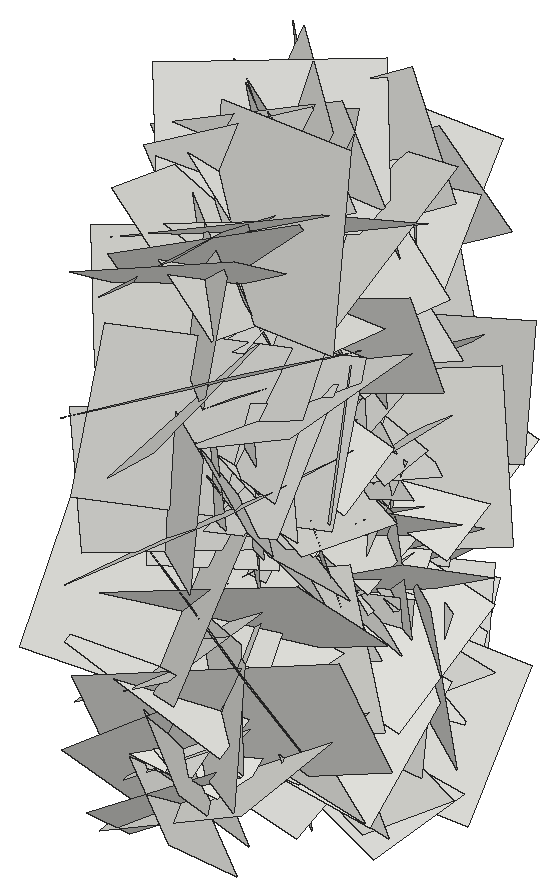
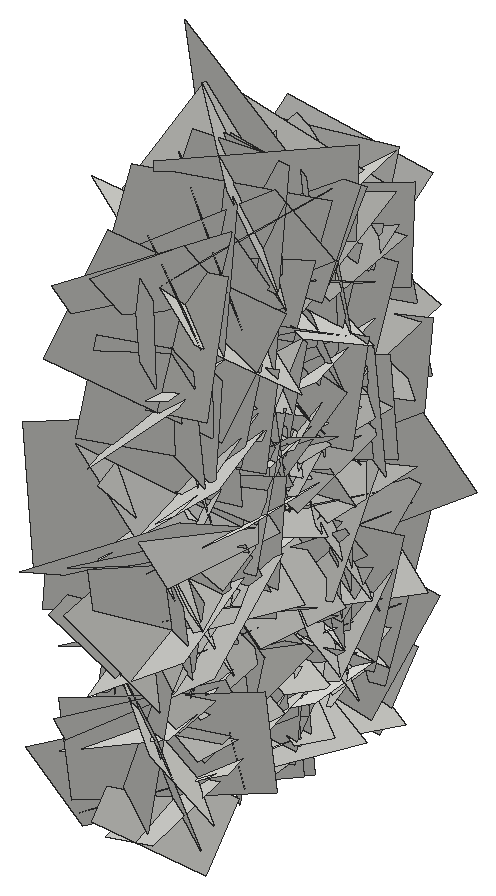
# SketchUp Ruby script. Lengths in inches.
U = 1.inch
M = Sketchup.active_model
def pt(a) = Geom::Point3d.new(a.map { |v| v * U })
def face(e, loops, mat)
  f = e.add_face(loops[0].map { |a| pt(a) })
  loops[1..].each { |l| e.add_face(l.map { |a| pt(a) }).erase! }
  f.material = f.back_material = mat if mat
  f
end
# faces: each face lists its corners as indices into pts; further lists are holes
def faces(e, pts, list, mat = nil) = list.each { |f| face(e, (f[0].is_a?(Array) ? f : [f]).map { |l| l.map { |i| pts[i] } }, mat) }
# xy, xz, yz: faces in a plane at the given z, y or x. An outline is a flat list of corners, or four numbers for a rectangle; further outlines are holes
def ring(l) = l.size == 4 ? [[l[0], l[1]], [l[2], l[1]], [l[2], l[3]], [l[0], l[3]]] : l.each_slice(2).to_a
def flat(e, list, mat, &to3) = list.each { |f| face(e, (f[0].is_a?(Array) ? f : [f]).map { |l| ring(l).map { |u, v| to3.(u, v) } }, mat) }
def xy(e, z, list, mat = nil) = flat(e, list, mat) { |x, y| [x, y, z] }
def xz(e, y, list, mat = nil) = flat(e, list, mat) { |x, z| [x, y, z] }
def yz(e, x, list, mat = nil) = flat(e, list, mat) { |y, z| [x, y, z] }
def lines(e, pts, list) = list.each { |a, b| e.add_line(pt(pts[a]), pt(pts[b])) }
# prism: a flat outline (further loops are holes) pulled along v
def prism(e, loops, v, mat = nil)
  f = face(e, loops, mat); d = Geom::Vector3d.new(v.map { |x| x * U })
  f.pushpull(f.normal.samedirection?(d) ? d.length : -d.length)
end
def box(e, o, s, mat = nil) = prism(e, [[o, [o[0] + s[0], o[1], o[2]], [o[0] + s[0], o[1] + s[1], o[2]], [o[0], o[1] + s[1], o[2]]]], [0, 0, s[2]], mat)
def at(x, y, z, deg = 0) = Geom::Transformation.translation(pt([x, y, z])) * Geom::Transformation.rotation(ORIGIN, Z_AXIS, deg.degrees)
def axes(o, x, y, z) = Geom::Transformation.new([*x, 0, *y, 0, *z, 0, *pt(o).to_a, 1])
def part(name) = M.definitions.add(name)
# library, detail: a bought-in or finely detailed component or shape, given as its bounding box
def library(name, o, s) = part(name).tap { |d| box(d.entities, o, s) }
def detail(e, o, s) = box(e.add_group.entities, o, s)
def put(e, d, t, mat = nil) = e.add_instance(d, t).tap { |i| i.material = mat if mat }
def group(e, t, mat = nil) = e.add_group.tap { |g| g.transformation = t; g.material = mat if mat }.entities
root = M.entities
c1 = part("Component\#6")
p = [[0.01,0,0],[0,3.24,4.54],[4.32,3.24,4.54],[4.33,0,0]]
faces(c1.entities,p,[[0,1,2,3]])
put(root,c1,axes([424.49,139.9,15.42],[-0.08068,-0.00169,-0.87701],[-0.08263,-0.87681,0.00845],[-0.92595,0.07839,0.07566]))
put(root,c1,axes([420.52,145.32,5.58],[0.01721,-0.24816,-0.73855],[-0.187,-0.7207,0.23828],[0.80443,-0.16223,0.07119]))
put(root,c1,axes([424.49,140.66,10.67],[0.05387,-0.70807,-1.02445],[0.25854,-0.99979,0.70312],[-1.29449,-0.22915,0.09779]))
put(root,c1,axes([424.49,141.11,17.69],[-0.01651,0.23078,-0.87547],[-0.12637,-0.8685,-0.22682],[-0.95135,0.11136,0.04532]))
put(root,c1,axes([420.52,138.56,10.4375],[-0.05239,0.37979,0.51244],[0.10197,0.51253,-0.37059],[0.66837,-0.04842,0.0967]))
put(root,c1,axes([424.49,149.05,6.52],[0.16475,-0.3536,-1.09271],[0.00842,-1.10231,0.35784],[-1.21738,-0.05548,-0.1454]))
put(root,c1,axes([424.49,142.09,4.39],[-0.13266,-0.06807,0.83796],[-0.05074,0.84639,0.06161],[-0.88972,-0.03812,-0.12846]))
put(root,c1,axes([424.49,136.25,6.15],[-0.02753,0.62765,0.83331],[0.11118,0.83092,-0.62258],[-1.10023,0.06826,-0.08377]))
put(root,c1,axes([420.52,141.82,12.65],[0.04235,0.31596,0.66399],[-0.14644,0.65635,-0.30401],[0.76557,0.10807,-0.09488]))
put(root,c1,axes([424.49,145.41,21.68],[-0.17174,-0.50133,-0.77339],[0.12403,-0.79008,0.48764],[-0.96905,-0.01227,0.19948]))
put(root,c1,axes([420.52,139.97,19.34],[-0.20036,-0.21311,0.82685],[-0.01235,0.84743,0.21575],[0.90502,-0.03562,0.186]))
put(root,c1,axes([424.49,135.11,11.54],[0.10699,0.00448,1.06975],[-0.01257,1.07444,-0.00338],[-1.13388,-0.01149,0.10098]))
put(root,c1,axes([420.52,141.75,2.2],[0.07408,-0.19814,0.56205],[0.01701,0.56632,0.19765],[0.63148,0.00798,-0.07126]))
put(root,c1,axes([424.49,137.79,2.1],[0.03475,-0.78477,0.75119],[0.11687,0.75006,0.77877],[-1.14558,0.05272,0.10224]))
put(root,c1,axes([420.52,139.2,5.38],[-0.02645,-0.5119,-0.36479],[0.13209,-0.36186,0.49927],[0.65307,0.05245,-0.11575]))
put(root,c1,axes([420.52,147.44,21.48],[0.11936,-0.32986,-0.48912],[-0.02265,-0.49991,0.33221],[0.62494,0.04489,0.10546]))
put(root,c1,axes([424.49,139.48,6.78],[-0.1397,0.74364,0.31774],[-0.04551,0.31504,-0.75514],[-0.85599,-0.13812,-0.01171]))
put(root,c1,axes([424.49,146.4375,4.35],[0.18242,-1.06895,0.55133],[0.10581,0.56772,1.06956],[-1.27052,-0.1062,0.16823]))
put(root,c1,axes([420.52,141.96,13.08],[0.07799,-0.57044,-0.33182],[-0.05167,-0.33766,0.56968],[0.69762,0.03877,0.07929]))
put(root,c1,axes([424.49,137.55,18.4],[0.05522,0.7917,0.38208],[-0.20111,0.38385,-0.76951],[-0.90986,-0.0368,0.19328]))
put(root,c1,axes([420.52,140.67,1.375],[0.09858,-0.02009,0.69473],[-0.09996,0.69407,0.03269],[0.72991,0.09776,-0.08935]))
put(root,c1,axes([420.52,143.63,3.63],[0.04495,-0.13338,0.65571],[0.00407,0.65706,0.13341],[0.70927,0.00468,-0.04233]))
put(root,c1,axes([420.52,139.35,17.19],[0.06054,-0.33637,0.61942],[-0.0607,0.61718,0.34043],[0.74468,0.07766,-0.02261]))
put(root,c1,axes([424.49,145.52,15.88],[0.20612,-0.51117,0.96001],[-0.04532,0.97089,0.52562],[-1.15198,-0.12966,0.1511]))
put(root,c1,axes([420.52,136.74,12.93],[0.11437,0.04247,0.59628],[0.02624,0.60507,-0.04758],[0.63311,-0.03275,-0.10574]))
put(root,c1,axes([420.52,142.73,15.75],[-0.26089,1.021,-0.12695],[-0.10549,-0.15355,-1.04195],[1.08548,0.23047,-0.13178]))
put(root,c1,axes([424.49,139.41,15.5],[-0.07329,-0.02436,0.98546],[0.16551,0.97513,0.03506],[-1.03171,0.15816,-0.06438]))
put(root,c1,axes([420.52,143.53,7.33],[-0.11895,-0.88372,0.009],[-0.0734,0.01784,0.88799],[0.93392,-0.11115,0.07094]))
put(root,c1,axes([424.49,142.07,24.73],[0.13514,0.30002,-0.93652],[-0.09595,-0.93677,-0.31242],[-1.03799,0.12565,-0.09305]))
put(root,c1,axes([420.52,138.58,20.36],[-0.30182,0.3301,1.08442],[-0.18064,1.09293,-0.37743],[1.1879,0.25007,0.21813]))
put(root,c1,axes([424.49,143.76,15.19],[-0.09057,0.86782,-0.29614],[0.1091,-0.28647,-0.86917],[-0.96584,-0.11373,-0.07041]))
put(root,c1,axes([424.49,139.77,3.95],[-0.11908,-0.78329,-0.0515],[-0.03618,-0.0471,0.79084],[-0.83129,0.11425,-0.02704]))
put(root,c1,axes([420.52,146.8125,4.55],[-0.17148,-0.83232,0.10491],[0.08015,0.09194,0.84603],[0.88562,-0.16948,-0.05625]))
put(root,c1,axes([424.49,145.52,18.22],[0.02537,0.1253,-0.85934],[-0.08829,-0.85537,-0.12704],[-0.91628,0.08589,-0.01155]))
put(root,c1,axes([424.49,143.66,16.18],[-0.1105,0.58717,-0.52568],[-0.01323,-0.53143,-0.59111],[-0.83529,-0.06926,0.0789]))
put(root,c1,axes([424.49,147.01,9.44],[0.18802,-1.10018,-0.17062],[0.06994,-0.16208,1.11371],[-1.17806,-0.18521,0.03889]))
put(root,c1,axes([420.52,143.33,2.25],[0.06381,-0.71847,0.0034],[-0.02834,0.00117,0.7205],[0.76106,0.06028,0.02655]))
put(root,c1,axes([424.49,144.05,16.5],[-0.02895,-0.76847,-0.41691],[0.01722,-0.41749,0.76847],[-0.92657,0.01625,0.02731]))
put(root,c1,axes([424.49,143.95,11.7],[0.02215,-0.88691,-0.38082],[0.08723,-0.37788,0.88459],[-1.0194,-0.05161,0.06742]))
put(root,c1,axes([420.52,147.56,10.64],[0.00206,-0.13591,-0.77504],[-0.03252,-0.77447,0.13573],[0.83344,-0.02988,0.00721]))
put(root,c1,axes([420.52,142.57,12.97],[-0.12959,-0.66136,0.5647],[0.03976,0.56572,0.67067],[0.92097,-0.11748,0.0505]))
put(root,c1,axes([424.49,141.85,18.04],[0.12661,-0.3078,1.12748],[0.24587,1.11705,0.28038],[-1.21422,0.1941,0.17434]))
put(root,c1,axes([420.52,147.06,19.23],[-0.16196,0.05609,-0.92604],[0.00217,-0.93849,-0.05718],[0.9834,0.01131,-0.15239]))
put(root,c1,axes([420.52,141.5625,11.54],[-0.13399,-0.80117,0.38482],[0.02481,0.38556,0.81039],[0.9418,-0.12414,0.0334]))
put(root,c1,axes([420.52,149.3125,5.88],[-0.15882,-0.57412,-0.80425],[-0.08368,-0.80389,0.58857],[1.04409,-0.15176,-0.07517]))
put(root,c1,axes([424.49,143.03,2.65],[0.18528,-0.93043,-0.12384],[-0.14778,-0.15031,0.9325],[-0.98392,-0.15263,-0.16338]))
put(root,c1,axes([420.52,141.35,5.69],[0.05421,0.52298,-0.48745],[0.04158,-0.49001,-0.52162],[0.75668,-0.01054,0.06359]))
put(root,c1,axes([424.49,145.65,3.28],[-0.1646,0.60158,-0.34623],[-0.0091,-0.35642,-0.61544],[-0.73568,-0.13018,0.08507]))
put(root,c1,axes([420.52,139.62,7.21],[-0.15609,-0.9187,-0.23757],[-0.00588,-0.23958,0.92989],[1.00583,-0.14396,-0.03143]))
put(root,c1,axes([420.52,143.17,8.1],[0.04482,0.75985,0.07181],[0.00358,0.07173,-0.76102],[0.80902,-0.04241,-0.00061]))
put(root,c1,axes([420.52,141.47,13.3125],[-0.15098,-0.93805,0.13539],[-0.00567,0.13771,0.94846],[1.00463,-0.1402,0.0257]))
put(root,c1,axes([424.49,139.94,18.75],[0.02341,-0.9115,0.17831],[0.09444,0.17962,0.90714],[-0.97996,-0.00447,0.09169]))
put(root,c1,axes([420.52,144.39,10.35],[-0.12238,0.87118,-0.30871],[-0.00416,-0.31157,-0.87778],[0.97971,0.1075,-0.04229]))
put(root,c1,axes([420.52,135.6875,17.375],[-0.11773,0.10526,0.9962],[-0.108,0.99592,-0.11659],[1.05635,0.11356,0.09911]))
put(root,c1,axes([420.52,136.7,5.12],[0.11008,0.58852,-0.4619],[-0.03608,-0.46213,-0.59646],[0.7922,-0.10282,0.03702]))
put(root,c1,axes([424.49,147.32,10.4375],[0.06119,-0.47987,-0.75245],[0.01649,-0.75336,0.48165],[-0.94584,-0.04418,-0.04028]))
put(root,c1,axes([420.52,147.32,10.4375],[-0.06119,-0.47987,-0.75245],[-0.01649,-0.75336,0.48165],[0.94584,-0.04418,-0.04028]))
put(root,c1,axes([424.49,136.7,5.12],[-0.11008,0.58852,-0.4619],[0.03608,-0.46213,-0.59646],[-0.7922,-0.10282,0.03702]))
put(root,c1,axes([424.49,135.6875,17.375],[0.11773,0.10526,0.9962],[0.108,0.99592,-0.11659],[-1.05635,0.11356,0.09911]))
put(root,c1,axes([424.49,144.39,10.35],[0.12238,0.87118,-0.30871],[0.00416,-0.31157,-0.87778],[-0.97971,0.1075,-0.04229]))
put(root,c1,axes([420.52,139.94,18.75],[-0.02341,-0.9115,0.17831],[-0.09444,0.17962,0.90714],[0.97996,-0.00447,0.09169]))
put(root,c1,axes([424.49,141.47,13.3125],[0.15098,-0.93805,0.13539],[0.00567,0.13771,0.94846],[-1.00463,-0.1402,0.0257]))
put(root,c1,axes([424.49,143.17,8.1],[-0.04482,0.75985,0.07181],[-0.00358,0.07173,-0.76102],[-0.80902,-0.04241,-0.00061]))
put(root,c1,axes([424.49,139.62,7.21],[0.15609,-0.9187,-0.23757],[0.00588,-0.23958,0.92989],[-1.00583,-0.14396,-0.03143]))
put(root,c1,axes([420.52,145.65,3.28],[0.1646,0.60158,-0.34623],[0.0091,-0.35642,-0.61544],[0.73568,-0.13018,0.08507]))
put(root,c1,axes([424.49,141.35,5.69],[-0.05421,0.52298,-0.48745],[-0.04158,-0.49001,-0.52162],[-0.75668,-0.01054,0.06359]))
put(root,c1,axes([420.52,143.03,2.65],[-0.18528,-0.93043,-0.12384],[0.14778,-0.15031,0.9325],[0.98392,-0.15263,-0.16338]))
put(root,c1,axes([424.49,149.3125,5.88],[0.15882,-0.57412,-0.80425],[0.08368,-0.80389,0.58857],[-1.04409,-0.15176,-0.07517]))
put(root,c1,axes([424.49,141.5625,11.54],[0.13399,-0.80117,0.38482],[-0.02481,0.38556,0.81039],[-0.9418,-0.12414,0.0334]))
put(root,c1,axes([424.49,147.06,19.23],[0.16196,0.05609,-0.92604],[-0.00217,-0.93849,-0.05718],[-0.9834,0.01131,-0.15239]))
put(root,c1,axes([420.52,141.85,18.04],[-0.12661,-0.3078,1.12748],[-0.24587,1.11705,0.28038],[1.21422,0.1941,0.17434]))
put(root,c1,axes([424.49,142.57,12.97],[0.12959,-0.66136,0.5647],[-0.03976,0.56572,0.67067],[-0.92097,-0.11748,0.0505]))
put(root,c1,axes([424.49,147.56,10.64],[-0.00206,-0.13591,-0.77504],[0.03252,-0.77447,0.13573],[-0.83344,-0.02988,0.00721]))
put(root,c1,axes([420.52,143.95,11.7],[-0.02215,-0.88691,-0.38082],[-0.08723,-0.37788,0.88459],[1.0194,-0.05161,0.06742]))
put(root,c1,axes([420.52,144.05,16.5],[0.02895,-0.76847,-0.41691],[-0.01722,-0.41749,0.76847],[0.92657,0.01625,0.02731]))
put(root,c1,axes([424.49,143.33,2.25],[-0.06381,-0.71847,0.0034],[0.02834,0.00117,0.7205],[-0.76106,0.06028,0.02655]))
put(root,c1,axes([420.52,147.01,9.44],[-0.18802,-1.10018,-0.17062],[-0.06994,-0.16208,1.11371],[1.17806,-0.18521,0.03889]))
put(root,c1,axes([420.52,143.66,16.18],[0.1105,0.58717,-0.52568],[0.01323,-0.53143,-0.59111],[0.83529,-0.06926,0.0789]))
put(root,c1,axes([420.52,145.52,18.22],[-0.02537,0.1253,-0.85934],[0.08829,-0.85537,-0.12704],[0.91628,0.08589,-0.01155]))
put(root,c1,axes([424.49,133.42,16.97],[0.14677,0.94615,0.46149],[0.22557,0.4307,-0.94687],[-1.09283,0.21597,-0.13346]))
put(root,c1,axes([424.49,146.8125,4.55],[0.17148,-0.83232,0.10491],[-0.08015,0.09194,0.84603],[-0.88562,-0.16948,-0.05625]))
put(root,c1,axes([420.52,139.77,3.95],[0.11908,-0.78329,-0.0515],[0.03618,-0.0471,0.79084],[0.83129,0.11425,-0.02704]))
put(root,c1,axes([420.52,143.76,15.19],[0.09057,0.86782,-0.29614],[-0.1091,-0.28647,-0.86917],[0.96584,-0.11373,-0.07041]))
put(root,c1,axes([424.49,138.58,20.36],[0.30182,0.3301,1.08442],[0.18064,1.09293,-0.37743],[-1.1879,0.25007,0.21813]))
put(root,c1,axes([420.52,142.07,24.73],[-0.13514,0.30002,-0.93652],[0.09595,-0.93677,-0.31242],[1.03799,0.12565,-0.09305]))
put(root,c1,axes([424.49,143.53,7.33],[0.11895,-0.88372,0.009],[0.0734,0.01784,0.88799],[-0.93392,-0.11115,0.07094]))
put(root,c1,axes([420.52,139.41,15.5],[0.07329,-0.02436,0.98546],[-0.16551,0.97513,0.03506],[1.03171,0.15816,-0.06438]))
put(root,c1,axes([424.49,142.73,15.75],[0.26089,1.021,-0.12695],[0.10549,-0.15355,-1.04195],[-1.08548,0.23047,-0.13178]))
put(root,c1,axes([424.49,136.74,12.93],[-0.11437,0.04247,0.59628],[-0.02624,0.60507,-0.04758],[-0.63311,-0.03275,-0.10574]))
put(root,c1,axes([420.52,145.52,15.88],[-0.20612,-0.51117,0.96001],[0.04532,0.97089,0.52562],[1.15198,-0.12966,0.1511]))
put(root,c1,axes([424.49,139.35,17.19],[-0.06054,-0.33637,0.61942],[0.0607,0.61718,0.34043],[-0.74468,0.07766,-0.02261]))
put(root,c1,axes([424.49,143.63,3.63],[-0.04495,-0.13338,0.65571],[-0.00407,0.65706,0.13341],[-0.70927,0.00468,-0.04233]))
put(root,c1,axes([424.49,140.67,1.375],[-0.09858,-0.02009,0.69473],[0.09996,0.69407,0.03269],[-0.72991,0.09776,-0.08935]))
put(root,c1,axes([420.52,137.55,18.4],[-0.05522,0.7917,0.38208],[0.20111,0.38385,-0.76951],[0.90986,-0.0368,0.19328]))
put(root,c1,axes([424.49,141.96,13.08],[-0.07799,-0.57044,-0.33182],[0.05167,-0.33766,0.56968],[-0.69762,0.03877,0.07929]))
put(root,c1,axes([420.52,146.4375,4.35],[-0.18242,-1.06895,0.55133],[-0.10581,0.56772,1.06956],[1.27052,-0.1062,0.16823]))
put(root,c1,axes([420.52,139.48,6.78],[0.1397,0.74364,0.31774],[0.04551,0.31504,-0.75514],[0.85599,-0.13812,-0.01171]))
put(root,c1,axes([424.49,147.44,21.48],[-0.11936,-0.32986,-0.48912],[0.02265,-0.49991,0.33221],[-0.62494,0.04489,0.10546]))
put(root,c1,axes([424.49,139.2,5.38],[0.02645,-0.5119,-0.36479],[-0.13209,-0.36186,0.49927],[-0.65307,0.05245,-0.11575]))
put(root,c1,axes([420.52,137.79,2.1],[-0.03475,-0.78477,0.75119],[-0.11687,0.75006,0.77877],[1.14558,0.05272,0.10224]))
put(root,c1,axes([424.49,141.75,2.2],[-0.07408,-0.19814,0.56205],[-0.01701,0.56632,0.19765],[-0.63148,0.00798,-0.07126]))
put(root,c1,axes([420.52,135.11,11.54],[-0.10699,0.00448,1.06975],[0.01257,1.07444,-0.00338],[1.13388,-0.01149,0.10098]))
put(root,c1,axes([424.49,139.97,19.34],[0.20036,-0.21311,0.82685],[0.01235,0.84743,0.21575],[-0.90502,-0.03562,0.186]))
put(root,c1,axes([420.52,145.41,21.68],[0.17174,-0.50133,-0.77339],[-0.12403,-0.79008,0.48764],[0.96905,-0.01227,0.19948]))
put(root,c1,axes([424.49,141.82,12.65],[-0.04235,0.31596,0.66399],[0.14644,0.65635,-0.30401],[-0.76557,0.10807,-0.09488]))
put(root,c1,axes([420.52,136.25,6.15],[0.02753,0.62765,0.83331],[-0.11118,0.83092,-0.62258],[1.10023,0.06826,-0.08377]))
put(root,c1,axes([420.52,142.09,4.39],[0.13266,-0.06807,0.83796],[0.05074,0.84639,0.06161],[0.88972,-0.03812,-0.12846]))
put(root,c1,axes([420.52,149.05,6.52],[-0.16475,-0.3536,-1.09271],[-0.00842,-1.10231,0.35784],[1.21738,-0.05548,-0.1454]))
put(root,c1,axes([424.49,138.56,10.4375],[0.05239,0.37979,0.51244],[-0.10197,0.51253,-0.37059],[-0.66837,-0.04842,0.0967]))
put(root,c1,axes([420.52,141.11,17.69],[0.01651,0.23078,-0.87547],[0.12637,-0.8685,-0.22682],[0.95135,0.11136,0.04532]))
put(root,c1,axes([420.52,140.66,10.67],[-0.05387,-0.70807,-1.02445],[-0.25854,-0.99979,0.70312],[1.29449,-0.22915,0.09779]))
put(root,c1,axes([424.49,145.32,5.58],[-0.01721,-0.24816,-0.73855],[0.187,-0.7207,0.23828],[-0.80443,-0.16223,0.07119]))
put(root,c1,axes([420.52,139.9,15.42],[0.08068,-0.00169,-0.87701],[0.08263,-0.87681,0.00845],[0.92595,0.07839,0.07566]))
put(root,c1,axes([424.49,139.99,14.29],[-0.01199,-0.16574,0.68191],[0.09091,0.67656,0.16586],[-0.73829,0.086,0.00935]))
put(root,c1,axes([424.49,147.58,14.43],[0.15626,-0.88067,0.15465],[0.14549,0.17716,0.87807],[-0.93656,-0.11942,0.1622]))
put(root,c1,axes([424.49,138.3,10.21],[0.07821,-0.14386,0.79141],[0.12147,0.78851,0.13265],[-0.84394,0.10016,0.09244]))
put(root,c1,axes([420.52,142.2,15.72],[-0.2001,0.61396,-1.10583],[-0.10306,-1.12181,-0.60624],[1.33676,0.00542,-0.21228]))
put(root,c1,axes([420.52,141.25,1.55],[0.11713,-0.0063,1.0149],[-0.13715,1.01248,0.02037],[1.06704,0.13083,-0.10878]))
put(root,c1,axes([420.52,144.34,6.82],[-0.01542,0.93301,-0.17325],[0.14993,-0.1692,-0.92309],[0.99466,0.03997,0.13646]))
put(root,c1,axes([420.52,137.99,14.66],[-0.08461,-0.27233,0.9902],[0.1352,0.98287,0.28059],[1.08015,-0.14435,0.04245]))
put(root,c1,axes([420.52,142.29,19.52],[0.02505,0.60517,0.90894],[-0.1077,0.90642,-0.60085],[1.15246,0.07156,-0.07591]))
put(root,c1,axes([420.52,144.58,9.97],[0.16827,0.58944,-0.69808],[-0.0398,-0.70373,-0.60275],[0.96765,-0.13145,0.0966]))
put(root,c1,axes([424.49,139.8125,20.98],[-0.02151,0.52563,-0.34386],[0.05265,-0.34162,-0.52514],[-0.66372,-0.04413,-0.03051]))
put(root,c1,axes([424.49,142.6,14.22],[0.18899,-0.6396,-0.42028],[-0.00285,-0.43205,0.65638],[-0.81124,-0.14749,-0.10022]))
put(root,c1,axes([424.49,145.36,10.15],[0.14636,-0.64891,0.3527],[0.01811,0.36152,0.65845],[-0.78267,-0.11298,0.08119]))
put(root,c1,axes([424.49,145.42,18.19],[0.07853,-0.05807,0.70782],[0.06912,0.70921,0.05136],[-0.74963,0.05931,0.07889]))
put(root,c1,axes([420.52,146.45,10.34],[0.10559,0.05407,-0.92917],[0.0532,-0.93343,-0.04894],[0.98516,0.04461,0.10223]))
put(root,c1,axes([424.49,141.95,12.73],[0.09992,0.55515,0.3498],[-0.02862,0.35638,-0.5583],[-0.69495,0.06514,0.07329]))
put(root,c1,axes([420.52,137.63,3.85],[-0.23328,-0.07655,1.22947],[0.08564,1.24535,0.092],[1.30295,-0.09556,0.21407]))
put(root,c1,axes([420.52,137.89,18.97],[0.02244,-0.79516,0.48934],[0.22215,0.48102,0.77258],[0.96443,-0.0923,-0.18934]))
put(root,c1,axes([424.49,139.18,13.74],[0.11062,-0.13563,-0.63299],[-0.03095,-0.6415,0.13263],[-0.6855,0.00708,-0.10814]))
put(root,c1,axes([420.52,141.92,3.18],[0.02887,1.0089,0.10446],[0.06921,0.10254,-1.00735],[1.07292,-0.03376,0.06217]))
put(root,c1,axes([420.52,138.34,13.4],[0.1901,0.66514,0.65147],[-0.02496,0.66648,-0.67398],[0.98658,-0.1113,-0.14258]))
put(root,c1,axes([420.52,138.76,9.15],[0.08107,-0.07376,-0.93469],[0.12107,-0.93007,0.08274],[0.98644,0.12021,0.06666]))
put(root,c1,axes([420.52,139.52,8.83],[0.01584,-0.12995,-1.07448],[0.00128,-1.07458,0.12998],[1.14724,0.003,0.01469]))
put(root,c1,axes([420.52,137.41,10.49],[0.17918,0.96529,0.20208],[-0.06958,0.21558,-0.97489],[1.04307,-0.15144,-0.09975]))
put(root,c1,axes([420.52,141.07,4.77],[-0.0925,1.07709,-0.24358],[0.13853,-0.23255,-1.07513],[1.16232,0.11343,0.10875]))
put(root,c1,axes([420.52,143.54,11.83],[-0.01207,0.98557,0.48784],[0.03058,0.48797,-0.98515],[1.16528,-0.0026,0.03091]))
put(root,c1,axes([424.49,142.82,6.12],[-0.04161,-0.60559,-0.03198],[0.13563,-0.03959,0.59276],[-0.62835,0.03156,0.13006]))
put(root,c1,axes([420.52,142.72,8.07],[-0.13823,0.05764,1.30603],[-0.0986,1.30878,-0.06705],[1.38223,0.09912,0.12583]))
put(root,c1,axes([420.52,138.64,15.1],[-0.05154,1.07135,-0.23626],[0.10153,-0.23144,-1.06922],[1.15847,0.06794,0.08319]))
put(root,c1,axes([420.52,138.49,4.97],[-0.13436,1.04009,0.6085],[0.04809,0.61554,-1.04268],[1.27641,0.08629,0.10334]))
put(root,c1,axes([424.49,137.29,3.46],[0.14224,0.61257,0.15159],[-0.04066,0.16261,-0.62315],[-0.66768,0.1206,0.07024]))
put(root,c1,axes([420.52,137.21,11.6875],[-0.11385,0.72886,-0.88593],[0.14818,-0.87485,-0.7367],[1.20699,0.17615,0.00688]))
put(root,c1,axes([420.52,143.17,19.13],[0.20193,0.9279,-0.28366],[0.04691,-0.29708,-0.94209],[1.02744,-0.16881,0.09877]))
put(root,c1,axes([420.52,142.88,1.98],[0.0351,0.64216,0.95117],[0.00533,0.95147,-0.64254],[1.21649,-0.02269,-0.02463]))
put(root,c1,axes([420.52,137.64,18.89],[0.26376,-0.64139,0.69016],[0.02251,0.71746,0.65911],[0.99845,0.15326,-0.19718]))
put(root,c1,axes([420.52,140.93,18.6875],[-0.10901,-0.41314,-1.06231],[0.28274,-1.04573,0.38087],[1.17466,0.21337,-0.19026]))
put(root,c1,axes([420.52,141.75,2.91],[-0.11729,-1.19784,-0.30033],[0.11289,-0.30967,1.19584],[1.30414,-0.08092,-0.13053]))
put(root,c1,axes([420.52,143.08,17.68],[-0.06532,-0.13436,-1.17102],[0.13166,-1.16683,0.12734],[1.24247,0.11658,-0.07506]))
put(root,c1,axes([420.52,140.04,10.48],[-0.03722,-1.27767,0.05021],[-0.04996,0.05148,1.27723],[1.35446,-0.03321,0.04849]))
put(root,c1,axes([420.52,140.59,7.56],[-0.03383,1.06332,0.50099],[0.10932,0.50178,-1.05842],[1.24115,-0.01522,0.10688]))
put(root,c1,axes([420.52,137.94,15.45],[-0.03401,0.89045,-0.73196],[0.17038,-0.72163,-0.88493],[1.2099,0.12665,0.10405]))
put(root,c1,axes([420.52,146.96,20.2],[-0.19126,-1.0536,-0.82739],[0.10265,-0.84293,1.05228],[1.41631,-0.08119,-0.188]))
put(root,c1,axes([420.52,139.77,22.87],[0.12093,1.26112,-0.05281],[-0.18505,-0.03675,-1.25475],[1.32509,-0.12022,-0.17041]))
put(root,c1,axes([420.52,139.44,14.86],[-0.04621,-1.16691,0.31838],[0.12643,0.31289,1.16311],[1.27589,-0.07327,-0.10372]))
put(root,c1,axes([420.52,141.48,7.17],[0.20337,0.82379,-0.77749],[-0.08888,-0.77608,-0.84298],[1.19742,-0.19752,0.06948]))
put(root,c1,axes([420.52,138.37,16.22],[0.07456,0.76169,-0.90937],[0.0504,-0.91204,-0.76025],[1.25638,-0.00862,0.08446]))
put(root,c1,axes([420.52,144.3,10.94],[0.16969,-0.07735,1.18237],[-0.06112,1.19119,0.08573],[1.2545,0.0685,-0.15576]))
put(root,c1,axes([420.52,144.73,5.33],[0.04426,-1.02294,0.56209],[0.16257,0.56238,1.01208],[1.2265,-0.03763,-0.15444]))
put(root,c1,axes([420.52,141.11,14.91],[0.10517,-0.78429,-0.79452],[0.18451,-0.77703,0.78876],[1.16892,0.19321,-0.05302]))
put(root,c1,axes([420.52,134.59,13.6],[0.14779,0.17555,1.29716],[-0.16453,1.29751,-0.15892],[1.37773,0.13612,-0.15813]))
put(root,c1,axes([420.52,148.13,7.79],[0.13698,0.11741,-1.23467],[-0.05668,-1.23967,-0.12348],[1.31343,-0.06574,0.12344]))
put(root,c1,axes([420.52,139.3125,6.46],[-0.05297,-0.89114,0.82127],[0.332,0.78454,0.87035],[1.24093,-0.24794,-0.1978]))
put(root,c1,axes([420.52,142.16,14.375],[-0.02255,-1.26636,-0.09652],[0.2141,-0.09868,1.25016],[1.3291,-0.00559,-0.20302]))
put(root,c1,axes([420.52,141.32,18.93],[-0.00931,-1.12138,0.55372],[0.26786,0.54072,1.09906],[1.29833,-0.1196,-0.22278]))
put(root,c1,axes([420.52,140.96,14.21],[0.1647,-0.56811,1.02456],[0.16232,1.03452,0.5504],[1.23116,-0.0604,-0.20963]))
put(root,c1,axes([420.52,137.06,3.09],[0.11239,-0.69918,1.17187],[0.18512,1.17269,0.68387],[1.43458,-0.09655,-0.18006]))
put(root,c1,axes([420.52,141.18,23.91],[0.20239,-0.45291,-1.29893],[0.24414,-1.28235,0.48098],[1.43758,0.28153,0.10118]))
